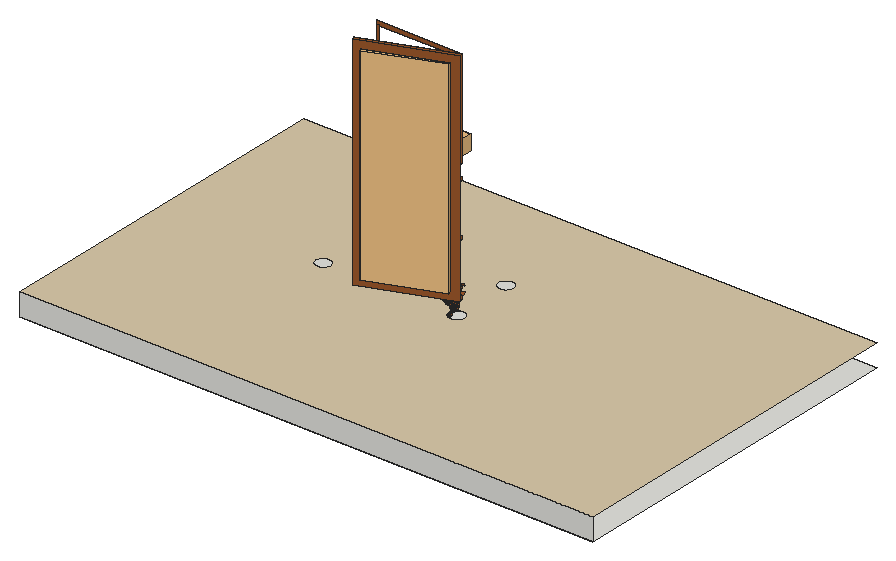
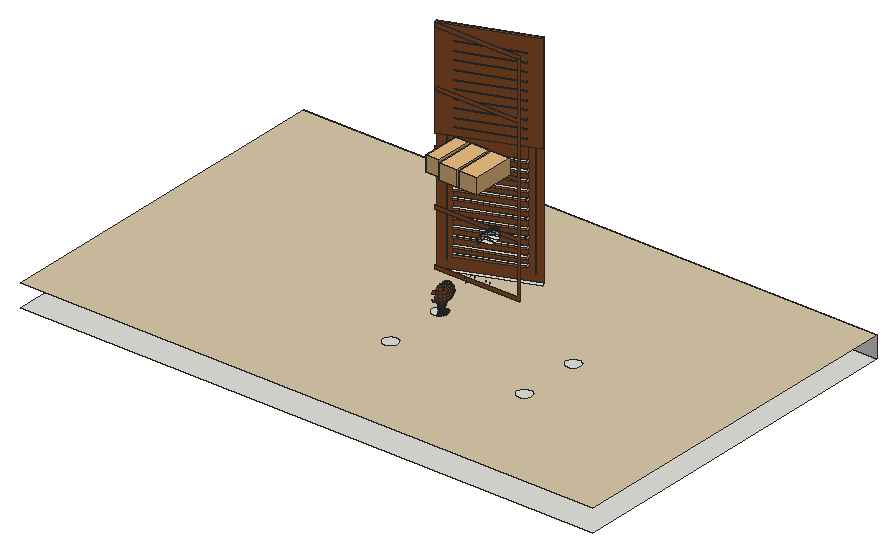
# SketchUp Ruby script. Lengths in inches.
U = 1.inch
M = Sketchup.active_model
def pt(a) = Geom::Point3d.new(a.map { |v| v * U })
def face(e, loops, mat)
  f = e.add_face(loops[0].map { |a| pt(a) })
  loops[1..].each { |l| e.add_face(l.map { |a| pt(a) }).erase! }
  f.material = f.back_material = mat if mat
  f
end
# faces: each face lists its corners as indices into pts; further lists are holes
def faces(e, pts, list, mat = nil) = list.each { |f| face(e, (f[0].is_a?(Array) ? f : [f]).map { |l| l.map { |i| pts[i] } }, mat) }
# xy, xz, yz: faces in a plane at the given z, y or x. An outline is a flat list of corners, or four numbers for a rectangle; further outlines are holes
def ring(l) = l.size == 4 ? [[l[0], l[1]], [l[2], l[1]], [l[2], l[3]], [l[0], l[3]]] : l.each_slice(2).to_a
def flat(e, list, mat, &to3) = list.each { |f| face(e, (f[0].is_a?(Array) ? f : [f]).map { |l| ring(l).map { |u, v| to3.(u, v) } }, mat) }
def xy(e, z, list, mat = nil) = flat(e, list, mat) { |x, y| [x, y, z] }
def xz(e, y, list, mat = nil) = flat(e, list, mat) { |x, z| [x, y, z] }
def yz(e, x, list, mat = nil) = flat(e, list, mat) { |y, z| [x, y, z] }
def lines(e, pts, list) = list.each { |a, b| e.add_line(pt(pts[a]), pt(pts[b])) }
# prism: a flat outline (further loops are holes) pulled along v
def prism(e, loops, v, mat = nil)
  f = face(e, loops, mat); d = Geom::Vector3d.new(v.map { |x| x * U })
  f.pushpull(f.normal.samedirection?(d) ? d.length : -d.length)
end
def box(e, o, s, mat = nil) = prism(e, [[o, [o[0] + s[0], o[1], o[2]], [o[0] + s[0], o[1] + s[1], o[2]], [o[0], o[1] + s[1], o[2]]]], [0, 0, s[2]], mat)
def at(x, y, z, deg = 0) = Geom::Transformation.translation(pt([x, y, z])) * Geom::Transformation.rotation(ORIGIN, Z_AXIS, deg.degrees)
def axes(o, x, y, z) = Geom::Transformation.new([*x, 0, *y, 0, *z, 0, *pt(o).to_a, 1])
def part(name) = M.definitions.add(name)
# library, detail: a bought-in or finely detailed component or shape, given as its bounding box
def library(name, o, s) = part(name).tap { |d| box(d.entities, o, s) }
def detail(e, o, s) = box(e.add_group.entities, o, s)
def put(e, d, t, mat = nil) = e.add_instance(d, t).tap { |i| i.material = mat if mat }
def group(e, t, mat = nil) = e.add_group.tap { |g| g.transformation = t; g.material = mat if mat }.entities
root = M.entities
M.materials.add("[Color K04]").color = [255, 50, 255]
M.materials.add("[Color L16]").color = [102, 0, 51]
M.materials.add("[Color M03]").color = [170, 170, 170]
M.materials.add("[Field Square Tile]").color = [217, 201, 169]
M.materials.add("[Wood Cherry Original]").color = [152, 86, 42]
c1 = library("shoe3",[0,0,0],[5.04,11.41,4.2])
c2 = part("Group\#13")
detail(c2.entities,[0,0,0],[19.875,0.8125,55.92])
c3 = library("Group\#9",[0,0,0],[6.05,17.1,6.94])
xy(root,0,[[118.75,0,274.48,96.25]])
xy(root,6,[[[118.75,0,274.48,96.25],[197.18,64.59,196.64,64.74,196.16,65.02,195.76,65.42,195.49,65.9,195.34,66.44,195.35,67,195.49,67.54,195.77,68.02,196.17,68.41,196.65,68.69,197.19,68.83,197.75,68.83,198.29,68.69,198.77,68.4,199.17,68.01,199.44,67.52,199.59,66.98,199.59,66.42,199.4375,65.89,199.16,65.4,198.76,65.01,198.28,64.73,197.74,64.59],[160.74,64.59,160.2,64.74,159.72,65.02,159.33,65.42,159.05,65.9,158.91,66.44,158.91,67,159.06,67.54,159.34,68.02,159.73,68.41,160.22,68.69,160.76,68.83,161.32,68.83,161.85,68.69,162.34,68.4,162.73,68.01,163.01,67.52,163.15,66.98,163.15,66.42,163,65.89,162.72,65.4,162.32,65.01,161.84,64.73,161.3,64.59],[160.74,47.97,160.2,48.11,159.72,48.4,159.33,48.79,159.05,49.28,158.91,49.82,158.91,50.375,159.06,50.91,159.34,51.4,159.73,51.79,160.22,52.07,160.76,52.21,161.32,52.21,161.85,52.06,162.34,51.78,162.73,51.38,163.01,50.9,163.15,50.36,163.15,49.8,163,49.26,162.72,48.78,162.32,48.39,161.84,48.11,161.3,47.97],[197.18,47.97,196.64,48.11,196.16,48.4,195.76,48.79,195.49,49.28,195.34,49.82,195.35,50.375,195.49,50.91,195.77,51.4,196.17,51.79,196.65,52.07,197.19,52.21,197.75,52.21,198.29,52.06,198.77,51.78,199.17,51.38,199.44,50.9,199.59,50.36,199.59,49.8,199.4375,49.26,199.16,48.78,198.76,48.39,198.28,48.11,197.74,47.97]]],"[Field Square Tile]")
xy(root,6,[[196.64,48.11,196.7,48.25,196.25,48.51,196.16,48.4],[196.16,48.4,196.25,48.51,195.88,48.88,195.76,48.79],[195.76,48.79,195.88,48.88,195.625,49.33,195.49,49.28],[195.49,49.28,195.625,49.33,195.49,49.84,195.34,49.82],[195.34,49.82,195.49,49.84,195.5,50.35,195.35,50.375],
  [195.5,50.35,195.63,50.85,195.49,50.91,195.35,50.375],[195.63,50.85,195.89,51.3,195.77,51.4,195.49,50.91],[195.89,51.3,196.26,51.67,196.17,51.79,195.77,51.4],[196.26,51.67,196.71,51.93,196.65,52.07,196.17,51.79]],"[Wood Cherry Original]")
xy(root,13.08,[[179.8,36.6,179.45,37.53,201.81,46.11,202.17,45.18]])
xy(root,16.73,[[183.07,37.85,198.59,43.81,198.23,44.74,182.72,38.79]],"[Wood Cherry Original]")
xy(root,17.26,[[183.07,37.85,182.72,38.79,198.23,44.74,198.59,43.81]])
xy(root,18.83,[[183.07,37.85,198.59,43.81,198.23,44.74,182.72,38.79]],"[Wood Cherry Original]")
xy(root,19.33,[[183.07,37.85,182.72,38.79,198.23,44.74,198.59,43.81]])
xy(root,21.15,[[183.07,37.85,198.59,43.81,198.23,44.74,182.72,38.79]],"[Wood Cherry Original]")
xy(root,21.65,[[183.07,37.85,182.72,38.79,198.23,44.74,198.59,43.81]])
xy(root,23.48,[[183.07,37.85,198.59,43.81,198.23,44.74,182.72,38.79]],"[Wood Cherry Original]")
xy(root,23.98,[[183.07,37.85,182.72,38.79,198.23,44.74,198.59,43.81]])
xy(root,25.8,[[183.07,37.85,198.59,43.81,198.23,44.74,182.72,38.79]],"[Wood Cherry Original]")
xy(root,26.3,[[183.07,37.85,182.72,38.79,198.23,44.74,198.59,43.81]])
xy(root,28.125,[[183.07,37.85,198.59,43.81,198.23,44.74,182.72,38.79]],"[Wood Cherry Original]")
xy(root,28.59,[[182.89,47.98,182.22,48.5,181.75,49.77,184.52,50.36,184.5,48.98,184,48.21]],"[Color K04]")
xy(root,28.625,[[183.07,37.85,182.72,38.79,198.23,44.74,198.59,43.81]])
xy(root,28.72,[[182.9,48.04,183.97,48.26,184.4375,49,182.27,48.54],[182.27,48.54,184.4375,49,184.46,50.35,181.81,49.78]])
xy(root,30.45,[[183.07,37.85,198.59,43.81,198.23,44.74,182.72,38.79]],"[Wood Cherry Original]")
xy(root,30.95,[[183.07,37.85,182.72,38.79,198.23,44.74,198.59,43.81]])
xy(root,32.78,[[183.07,37.85,198.59,43.81,198.23,44.74,182.72,38.79]],"[Wood Cherry Original]")
xy(root,33.28,[[183.07,37.85,182.72,38.79,198.23,44.74,198.59,43.81]])
xy(root,35.1,[[183.07,37.85,198.59,43.81,198.23,44.74,182.72,38.79]],"[Wood Cherry Original]")
xy(root,35.6,[[183.07,37.85,182.72,38.79,198.23,44.74,198.59,43.81]])
xy(root,37.43,[[183.07,37.85,198.59,43.81,198.23,44.74,182.72,38.79]],"[Wood Cherry Original]")
xy(root,37.93,[[183.07,37.85,182.72,38.79,198.23,44.74,198.59,43.81]])
xy(root,39.75,[[183.07,37.85,198.59,43.81,198.23,44.74,182.72,38.79]],"[Wood Cherry Original]")
xy(root,40.25,[[183.07,37.85,182.72,38.79,198.23,44.74,198.59,43.81]])
xy(root,42.08,[[183.07,37.85,198.59,43.81,198.23,44.74,182.72,38.79]],"[Wood Cherry Original]")
xy(root,42.58,[[183.07,37.85,182.72,38.79,198.23,44.74,198.59,43.81]])
xy(root,47.97,[[183.07,37.85,198.59,43.81,198.23,44.74,182.72,38.79]],"[Wood Cherry Original]")
xy(root,48.47,[[183.07,37.85,182.72,38.79,198.23,44.74,198.59,43.81]])
xy(root,50.29,[[183.07,37.85,198.59,43.81,198.23,44.74,182.72,38.79]],"[Wood Cherry Original]")
xy(root,50.79,[[183.07,37.85,182.72,38.79,198.23,44.74,198.59,43.81]])
xy(root,52.62,[[183.07,37.85,198.59,43.81,198.23,44.74,182.72,38.79]],"[Wood Cherry Original]")
xy(root,53.12,[[183.07,37.85,182.72,38.79,198.23,44.74,198.59,43.81]])
xy(root,54.94,[[183.07,37.85,198.59,43.81,198.23,44.74,182.72,38.79]],"[Wood Cherry Original]")
xy(root,55.44,[[183.07,37.85,182.72,38.79,198.23,44.74,198.59,43.81]])
xy(root,57.27,[[183.07,37.85,198.59,43.81,198.23,44.74,182.72,38.79]],"[Wood Cherry Original]")
xy(root,57.77,[[183.07,37.85,182.72,38.79,198.23,44.74,198.59,43.81]])
xy(root,59.59,[[183.07,37.85,198.59,43.81,198.23,44.74,182.72,38.79]],"[Wood Cherry Original]")
xy(root,60.09,[[183.07,37.85,182.72,38.79,198.23,44.74,198.59,43.81]])
xy(root,61.92,[[183.07,37.85,198.59,43.81,198.23,44.74,182.72,38.79]],"[Wood Cherry Original]")
xy(root,62.42,[[183.07,37.85,182.72,38.79,198.23,44.74,198.59,43.81]])
xy(root,64.24,[[183.07,37.85,198.59,43.81,198.23,44.74,182.72,38.79]],"[Wood Cherry Original]")
xy(root,64.74,[[183.07,37.85,182.72,38.79,198.23,44.74,198.59,43.81]])
xy(root,66.57,[[183.07,37.85,198.59,43.81,198.23,44.74,182.72,38.79]],"[Wood Cherry Original]")
xy(root,67.07,[[183.07,37.85,182.72,38.79,198.23,44.74,198.59,43.81]])
xy(root,68.89,[[183.07,37.85,198.59,43.81,198.23,44.74,182.72,38.79]],"[Wood Cherry Original]")
xy(root,69.39,[[183.07,37.85,182.72,38.79,198.23,44.74,198.59,43.81]])
xy(root,73.08,[[179.8,36.6,202.17,45.18,201.81,46.11,179.45,37.53]],"[Wood Cherry Original]")
xz(root,0,[[118.75,0,274.48,6]])
xz(root,46.11,[[178.85,13.08,201.81,13.08,201.81,14.08,179.35,14.08,179.35,27.58,201.81,27.58,201.81,28.58,179.35,28.58,179.35,42.08,201.81,42.08,201.81,43.08,179.35,43.08,179.35,56.58,201.81,56.58,201.81,57.58,179.35,57.58,179.35,72.08,178.85,72.08],[178.85,72.08,201.81,73.08]],"[Wood Cherry Original]")
yz(root,195.97,[[49.9,8.1,50.29,8.4]],"[Wood Cherry Original]")
yz(root,196.27,[[49.93,6.79,50.25,6.94]],"[Wood Cherry Original]")
p = [[196.34,48.63,6.03],[196.25,48.51,6],[196.7,48.25,6],[196.76,48.39,6.03],[196.43,48.75,6.08],[196.81,48.52,6.08],
  [196,48.97,6.03],[195.88,48.88,6],[196.12,49.06,6.08],[195.76,49.39,6.03],[195.625,49.33,6],[195.9,49.44,6.08],
  [195.64,49.85,6.03],[195.49,49.84,6],[195.78,49.87,6.08],[195.64,50.33,6.03],[195.5,50.35,6],[195.78,50.32,6.08],
  [195.77,50.8,6.03],[195.63,50.85,6],[195.9,50.74,6.08],[196.125,51.125,6.08],[196.01,51.21,6.03],[195.89,51.3,6],
  [196.4375,51.4375,6.08],[196.35,51.55,6.03],[196.26,51.67,6],[196.82,51.66,6.08],[196.77,51.79,6.03],[196.71,51.93,6],
  [196.51,48.85,6.16],[196.86,48.64,6.16],[196.22,49.14,6.16],[196.02,49.49,6.16],[195.91,49.89,6.16],[195.91,50.3,6.16],
  [196.02,50.69,6.16],[196.23,51.05,6.16],[196.52,51.33,6.16],[196.87,51.54,6.16],[196.58,48.94,6.25],[196.91,48.75,6.25],
  [196.3125,49.21,6.25],[196.125,49.54,6.25],[196.03,49.9,6.25],[196.03,50.28,6.25],[196.13,50.65,6.25],[196.32,50.97,6.25],
  [196.59,51.24,6.25],[196.92,51.43,6.25],[196.64,49.02,6.37],[196.94,48.84,6.37],[196.39,49.27,6.37],[196.21,49.57,6.37],
  [196.12,49.92,6.37],[196.125,50.27,6.37],[196.22,50.61,6.37],[196.39,50.92,6.37],[196.65,51.16,6.37],[196.95,51.34,6.37],
  [196.68,49.08,6.5],[196.97,48.91,6.5],[196.45,49.3125,6.5],[196.28,49.6,6.5],[196.2,49.93,6.5],[196.2,50.26,6.5],
  [196.29,50.58,6.5],[196.45,50.87,6.5],[196.69,51.1,6.5],[196.98,51.27,6.5],[196.49,49.34,6.64],[196.71,49.12,6.64],
  [196.33,49.62,6.64],[196.25,49.93,6.64],[196.25,50.25,6.64],[196.33,50.5625,6.64],[196.49,50.84,6.64],[196.72,51.0625,6.64],
  [196.51,49.36,6.79],[196.73,49.14,6.79],[196.35,49.63,6.79],[196.27,49.93,6.79],[196.27,50.25,6.79],[196.36,50.55,6.79],
  [196.51,50.82,6.79],[196.74,51.04,6.79],[196.51,49.36,6.94],[196.73,49.14,6.94],[196.35,49.63,6.94],[196.27,49.93,6.94],
  [196.36,50.55,6.94],[196.27,50.25,6.94],[196.51,50.82,6.94],[196.74,51.04,6.94],[196.49,49.34,7.09],[196.71,49.12,7.09],
  [196.33,49.62,7.09],[196.25,49.93,7.09],[196.25,50.25,7.09],[196.33,50.5625,7.09],[196.49,50.84,7.09],[196.72,51.06,7.09],
  [196.45,49.3125,7.23],[196.68,49.07,7.23],[196.28,49.6,7.23],[196.2,49.92,7.23],[196.2,50.26,7.23],[196.28,50.58,7.23],
  [196.45,50.87,7.23],[196.69,51.11,7.23],[196.61,48.99,7.51],[196.97,48.91,7.23],[196.93,48.8,7.51],[196.36,49.24,7.51],
  [196.18,49.56,7.51],[196.09,49.91,7.51],[196.09,50.27,7.51],[196.18,50.625,7.51],[196.36,50.9375,7.51],[196.62,51.19,7.51],
  [196.9375,51.375,7.51],[196.98,51.27,7.23],[196.57,48.93,7.8],[196.9,48.73,7.8],[196.3,49.2,7.8],[196.11,49.53,7.8],
  [196.01,49.9,7.8],[196.01,50.28,7.8],[196.11,50.65,7.8],[196.3,50.98,7.8],[196.58,51.25,7.8],[196.91,51.45,7.8],
  [196.54,48.89,8.1],[196.88,48.7,8.1],[196.27,49.17,8.1],[196.07,49.52,8.1],[195.97,49.9,8.1],[195.97,50.29,8.1],
  [196.08,50.67,8.1],[196.27,51.01,8.1],[196.55,51.29,8.1],[196.89,51.48,8.1],[196.54,48.89,8.4],[196.88,48.69,8.4],
  [196.26,49.17,8.4],[196.07,49.51,8.4],[195.97,49.9,8.4],[196.07,50.67,8.4],[195.97,50.29,8.4],[196.27,51.01,8.4],
  [196.55,51.29,8.4],[196.89,51.48,8.4],[196.5625,48.92,8.7],[196.9,48.73,8.7],[196.29,49.19,8.7],[196.1,49.53,8.7],
  [196,49.9,8.7],[196,50.29,8.7],[196.1,50.66,8.7],[196.3,50.99,8.7],[196.57,51.26,8.7],[196.91,51.45,8.7],
  [196.61,48.98,8.99],[196.92,48.79,8.99],[196.35,49.24,8.99],[196.16,49.55,8.99],[196.07,49.91,8.99],[196.07,50.28,8.99],
  [196.17,50.63,8.99],[196.35,50.95,8.99],[196.61,51.21,8.99],[196.93,51.39,8.99],[196.18,48.42,9.21],[196.65,48.14,9.21],
  [195.79,48.81,9.21],[195.52,49.29,9.21],[195.375,49.82,9.21],[195.375,50.37,9.21],[195.52,50.9,9.21],[195.8,51.375,9.21],
  [196.1875,51.76,9.21],[196.67,52.04,9.21],[195.82,47.96,9.66],[196.43,47.61,9.66],[195.33,48.46,9.66],[194.98,49.07,9.66],
  [194.8,49.75,9.66],[194.8,50.45,9.66],[194.99,51.125,9.66],[195.34,51.73,9.66],[195.84,52.23,9.66],[196.45,52.57,9.66],
  [196.28,47.26,10.28],[197.1,47.42,9.66],[197.05,47.05,10.28],[195.59,47.66,10.28],[195.02,48.23,10.28],[194.63,48.92,10.28],
  [194.42,49.7,10.28],[194.43,50.5,10.28],[194.64,51.27,10.28],[195.04,51.96,10.28],[195.61,52.53,10.28],[196.3,52.93,10.28],
  [197.08,53.13,10.28],[197.125,52.75,9.66],[196.23,47.14,11],[197.04,46.92,11],[195.51,47.56,11],[194.92,48.15,11],
  [194.5,48.875,11],[194.29,49.68,11],[194.29,50.52,11],[194.51,51.32,11],[194.93,52.04,11],[195.53,52.63,11],
  [196.25,53.05,11],[196.28,47.26,11.72],[197.05,47.05,11.72],[195.59,47.66,11.72],[195.02,48.23,11.72],[194.63,48.92,11.72],
  [194.42,49.7,11.72],[194.43,50.5,11.72],[194.64,51.27,11.72],[195.04,51.96,11.72],[195.61,52.53,11.72],[196.3,52.93,11.72],
  [196.43,47.61,12.34],[197.1,47.42,12.34],[195.82,47.96,12.34],[195.33,48.46,12.34],[194.98,49.07,12.34],[194.8,49.75,12.34],
  [194.8,50.45,12.34],[194.99,51.125,12.34],[195.34,51.73,12.34],[195.84,52.23,12.34],[196.45,52.57,12.34],[197.125,52.75,12.34],
  [197.08,53.13,11.72],[196.18,48.42,12.79],[196.65,48.14,12.79],[195.79,48.81,12.79],[195.52,49.29,12.79],[195.375,49.82,12.79],
  [195.375,50.37,12.79],[195.52,50.9,12.79],[195.8,51.375,12.79],[196.1875,51.76,12.79],[196.67,52.04,12.79],[196.61,48.98,13.01],
  [196.92,48.79,13.01],[196.35,49.24,13.01],[196.16,49.55,13.01],[196.07,49.91,13.01],[196.07,50.28,13.01],[196.17,50.63,13.01],
  [196.35,50.95,13.01],[196.61,51.21,13.01],[196.93,51.39,13.01],[196.93,49.68,12.97],[197.05,49.56,12.97],[196.84,49.83,12.97],
  [196.8,50,12.97],[196.8,50.18,12.97],[196.85,50.35,12.97],[196.93,50.5,12.97],[197.06,50.62,12.97],[179.8,36.6,13.08],
  [202.17,45.18,13.08],[202.17,45.18,73.08],[179.8,36.6,73.08],[198.59,43.81,16.73],[183.07,37.85,16.73],[183.07,37.85,17.26],
  [183.07,37.85,18.83],[183.07,37.85,19.33],[183.07,37.85,21.15],[183.07,37.85,21.65],[183.07,37.85,23.48],[183.07,37.85,23.98],
  [183.07,37.85,25.8],[183.07,37.85,26.3],[183.07,37.85,28.125],[183.07,37.85,28.625],[183.07,37.85,30.45],[183.07,37.85,30.95],
  [183.07,37.85,32.78],[183.07,37.85,33.28],[183.07,37.85,35.1],[183.07,37.85,35.6],[183.07,37.85,37.43],[183.07,37.85,37.93],
  [183.07,37.85,39.75],[183.07,37.85,40.25],[183.07,37.85,42.08],[183.07,37.85,42.58],[183.07,37.85,47.97],[183.07,37.85,48.47],
  [183.07,37.85,50.29],[183.07,37.85,50.79],[183.07,37.85,52.62],[183.07,37.85,53.12],[183.07,37.85,54.94],[183.07,37.85,55.44],
  [183.07,37.85,57.27],[183.07,37.85,57.77],[183.07,37.85,59.59],[183.07,37.85,60.09],[183.07,37.85,61.92],[183.07,37.85,62.42],
  [183.07,37.85,64.24],[183.07,37.85,64.74],[183.07,37.85,66.57],[183.07,37.85,67.07],[183.07,37.85,68.89],[183.07,37.85,69.39],
  [198.59,43.81,69.39],[198.59,43.81,68.89],[198.59,43.81,67.07],[198.59,43.81,66.57],[198.59,43.81,64.74],[198.59,43.81,64.24],
  [198.59,43.81,62.42],[198.59,43.81,61.92],[198.59,43.81,60.09],[198.59,43.81,59.59],[198.59,43.81,57.77],[198.59,43.81,57.27],
  [198.59,43.81,55.44],[198.59,43.81,54.94],[198.59,43.81,53.12],[198.59,43.81,52.62],[198.59,43.81,50.79],[198.59,43.81,50.29],
  [198.59,43.81,48.47],[198.59,43.81,47.97],[198.59,43.81,42.58],[198.59,43.81,42.08],[198.59,43.81,40.25],[198.59,43.81,39.75],
  [198.59,43.81,37.93],[198.59,43.81,37.43],[198.59,43.81,35.6],[198.59,43.81,35.1],[198.59,43.81,33.28],[198.59,43.81,32.78],
  [198.59,43.81,30.95],[198.59,43.81,30.45],[198.59,43.81,28.625],[198.59,43.81,28.125],[198.59,43.81,26.3],[198.59,43.81,25.8],
  [198.59,43.81,23.98],[198.59,43.81,23.48],[198.59,43.81,21.65],[198.59,43.81,21.15],[198.59,43.81,19.33],[198.59,43.81,18.83],
  [198.59,43.81,17.26],[182.72,38.79,16.73],[182.72,38.79,17.26],[188.82,52.19,17.8125],[188.82,52.2,17.86],[188.78,52.07,18],
  [188.78,51.96,16.99],[188.78,51.95,16.83],[188.78,51.97,16.9],[188.78,52.09,18.17],[188.82,52.23,18.19],[188.84,52.25,17.82],
  [183.02,51.03,18.4],[182.99,51.04,18.23],[183.02,51.02,18.23],[184.19,51.03,18.4],[184.1875,51.02,18.23],[184.22,51.04,18.23],
  [186.99,51.03,18.4],[186.96,51.04,18.23],[186.99,51.02,18.23],[188.15,51.03,18.4],[188.16,51.02,18.23],[188.1875,51.04,18.23],
  [182.72,38.79,18.83],[182.72,38.79,19.33],[182.72,38.79,21.15],[182.72,38.79,21.65],[182.72,38.79,23.48],[182.72,38.79,23.98],
  [182.72,38.79,25.8],[182.72,38.79,26.3],[182.72,38.79,28.125],[182.72,38.79,28.625],[182.89,47.98,28.59],[182.87,47.89,28.67],
  [182.13,48.48,28.67],[184,48.21,28.59],[184.05,48.14,28.67],[184.5,48.98,28.59],[184.59,49,28.67],[184.52,50.36,28.59],
  [184.6,50.375,28.67],[181.58,51.11,28.65],[184.32,51.48,28.65],[184.18,52.65,28.74],[184.1,52.64,28.66],[184.07,53.66,28.58],
  [182.87,47.89,28.96],[184.05,48.14,28.96],[182.9,48.03,29.63],[182.9,48.04,28.72],[182.27,48.54,28.72],[183.97,48.26,29.63],
  [183.97,48.26,28.72],[184.59,49,28.96],[184.375,49.1,29.625],[184.4375,49,28.72],[184.38,50.39,29.53],[184.46,50.35,28.72],
  [184.6,50.375,28.96],[181.63,51.12,28.78],[181.81,49.78,28.72],[184.27,51.47,28.78],[184.29,51.46,29.46],[184.4,51.49,28.73],
  [184.4,51.49,28.96],[181.45,52.22,28.66],[184.18,52.65,28.96],[184.05,52.64,28.79],[181.51,52.23,28.79],[184.15,52.65,29.4],
  [184.17,53.7,29.36],[182.86,47.9,29.65],[184.06,48.15,29.65],[184.51,49.0625,29.65],[184.52,50.4,29.55],[184.43,51.47,29.47],
  [184.29,52.66,29.38],[184.3125,53.69,29.34],[184.19,52.7,29.96],[184.33,52.7,29.97],[184.22,53.7,29.89],[184.36,53.7,29.89],
  [184.21,50.36,30.17],[184.2,51.51,30.06],[184.34,51.52,30.09],[182.14,48.51,29.65],[182.9,48.04,30.32],[183.8,48.21,30.32],
  [182.93,48.17,30.28],[182.26,48.59,29.63],[183.73,48.32,30.27],[184.25,49.08,30.32],[184.13,49.11,30.25],[184.34,50.37,30.23],
  [184.13,52.74,30.47],[184.27,52.74,30.55],[184.01,51.56,30.57],[184.11,51.56,30.68],[183.9,50.41,30.65],[183.97,50.41,30.79],
  [182.27,48.6,30.32],[182.93,48.29,30.9],[183.51,48.4,30.9],[182.97,48.38,30.78],[182.38,48.68,30.28],[183.47,48.48,30.77],
  [183.77,49.23,30.9],[183.72,49.25,30.76],[182.6,48.79,30.78],[182.72,38.79,30.45],[182.72,38.79,30.95],[184.04,51.56,30.65],
  [184.1875,52.75,30.54],[183.91,50.41,30.74],[183.72,49.25,30.84],[182.58,48.78,30.86],[182.95,48.35,30.87],[183.47,48.45,30.86],
  [182.51,48.74,30.9],[182.72,38.79,32.78],[182.72,38.79,33.28],[182.72,38.79,35.1],[182.72,38.79,35.6],[182.72,38.79,37.43],
  [182.72,38.79,37.93],[182.72,38.79,39.75],[182.72,38.79,40.25],[182.72,38.79,42.08],[182.72,38.79,42.58],[201.81,46.11,56.58],
  [201.81,46.11,46.26],[179.45,37.53,46.26],[179.45,37.53,73.08],[201.81,46.11,73.08],[201.81,46.11,72.08],[201.81,46.11,57.58],
  [182.72,38.79,69.39],[182.72,38.79,68.89],[198.23,44.74,68.89],[198.23,44.74,69.39],[182.72,38.79,67.07],[182.72,38.79,66.57],
  [198.23,44.74,66.57],[198.23,44.74,67.07],[182.72,38.79,64.74],[182.72,38.79,64.24],[198.23,44.74,64.24],[198.23,44.74,64.74],
  [182.72,38.79,62.42],[182.72,38.79,61.92],[198.23,44.74,61.92],[198.23,44.74,62.42],[182.72,38.79,60.09],[182.72,38.79,59.59],
  [198.23,44.74,59.59],[198.23,44.74,60.09],[182.72,38.79,57.77],[182.72,38.79,57.27],[198.23,44.74,57.27],[198.23,44.74,57.77],
  [182.72,38.79,55.44],[182.72,38.79,54.94],[198.23,44.74,54.94],[198.23,44.74,55.44],[182.72,38.79,53.12],[182.72,38.79,52.62],
  [198.23,44.74,52.62],[198.23,44.74,53.12],[182.72,38.79,50.79],[182.72,38.79,50.29],[198.23,44.74,50.29],[198.23,44.74,50.79],
  [182.72,38.79,48.47],[182.72,38.79,47.97],[198.23,44.74,47.97],[198.23,44.74,48.47]]
faces(root,p,[[0,1,2,3],[4,0,3,5],[6,7,1,0],[8,6,0,4],[9,10,7,6],[11,9,6,8],[12,13,10,9],[14,12,9,11],
  [15,16,13,12],[17,15,12,14],[18,19,16,15],[20,18,15,17],[21,22,18,20],[22,23,19,18],[24,25,22,21],[25,26,23,22],
  [27,28,25,24],[28,29,26,25],[30,4,5,31],[32,8,4,30],[33,11,8,32],[34,14,11,33],[35,17,14,34],[36,20,17,35],
  [37,21,20,36],[38,24,21,37],[39,27,24,38],[40,30,31,41],[42,32,30,40],[43,33,32,42],[44,34,33,43],[45,35,34,44],
  [46,36,35,45],[47,37,36,46],[48,38,37,47],[49,39,38,48],[50,40,41,51],[52,42,40,50],[53,43,42,52],[54,44,43,53],
  [55,45,44,54],[56,46,45,55],[57,47,46,56],[58,48,47,57],[59,49,48,58],[60,50,51,61],[62,52,50,60],[63,53,52,62],
  [64,54,53,63],[65,55,54,64],[66,56,55,65],[67,57,56,66],[68,58,57,67],[69,59,58,68],[70,62,60,71],[72,63,62,70],
  [73,64,63,72],[74,65,64,73],[75,66,65,74],[76,67,66,75],[77,68,67,76],[78,70,71,79],[80,72,70,78],[81,73,72,80],
  [82,74,73,81],[83,75,74,82],[84,76,75,83],[85,77,76,84],[86,78,79,87],[88,80,78,86],[89,81,80,88],[90,83,82,91],
  [92,84,83,90],[93,85,84,92],[94,86,87,95],[96,88,86,94],[97,89,88,96],[98,91,89,97],[99,90,91,98],[100,92,90,99],
  [101,93,92,100],[102,94,95,103],[104,96,94,102],[105,97,96,104],[106,98,97,105],[107,99,98,106],[108,100,99,107],[109,101,100,108],
  [110,103,111,112],[113,102,103,110],[114,104,102,113],[115,105,104,114],[116,106,105,115],[117,107,106,116],[118,108,107,117],[119,109,108,118],
  [120,121,109,119],[122,110,112,123],[124,113,110,122],[125,114,113,124],[126,115,114,125],[127,116,115,126],[128,117,116,127],[129,118,117,128],
  [130,119,118,129],[131,120,119,130],[132,122,123,133],[134,124,122,132],[135,125,124,134],[136,126,125,135],[137,127,126,136],[138,128,127,137],
  [139,129,128,138],[140,130,129,139],[141,131,130,140],[142,132,133,143],[144,134,132,142],[145,135,134,144],[146,136,135,145],[147,138,137,148],
  [149,139,138,147],[150,140,139,149],[151,141,140,150],[152,142,143,153],[154,144,142,152],[155,145,144,154],[156,146,145,155],[157,148,146,156],
  [158,147,148,157],[159,149,147,158],[160,150,149,159],[161,151,150,160],[162,152,153,163],[164,154,152,162],[165,155,154,164],[166,156,155,165],
  [167,157,156,166],[168,158,157,167],[169,159,158,168],[170,160,159,169],[171,161,160,170],[172,162,163,173],[174,164,162,172],[175,165,164,174],
  [176,166,165,175],[177,167,166,176],[178,168,167,177],[179,169,168,178],[180,170,169,179],[181,171,170,180],[182,172,173,183],[184,174,172,182],
  [185,175,174,184],[186,176,175,185],[187,177,176,186],[188,178,177,187],[189,179,178,188],[190,180,179,189],[191,181,180,190],[192,183,193,194],
  [195,182,183,192],[196,184,182,195],[197,185,184,196],[198,186,185,197],[199,187,186,198],[200,188,187,199],[201,189,188,200],[202,190,189,201],
  [203,191,190,202],[204,205,191,203],[206,192,194,207],[208,195,192,206],[209,196,195,208],[210,197,196,209],[211,198,197,210],[212,199,198,211],
  [213,200,199,212],[214,201,200,213],[215,202,201,214],[216,203,202,215],[217,206,207,218],[219,208,206,217],[220,209,208,219],[221,210,209,220],
  [222,211,210,221],[223,212,211,222],[224,213,212,223],[225,214,213,224],[226,215,214,225],[227,216,215,226],[228,217,218,229],[230,219,217,228],
  [231,220,219,230],[232,221,220,231],[233,222,221,232],[234,223,222,233],[235,224,223,234],[236,225,224,235],[237,226,225,236],[238,227,226,237],
  [239,240,227,238],[241,230,228,242],[243,231,230,241],[244,232,231,243],[245,233,232,244],[246,234,233,245],[247,235,234,246],[248,236,235,247],
  [249,237,236,248],[250,238,237,249],[251,241,242,252],[253,243,241,251],[254,244,243,253],[255,245,244,254],[256,246,245,255],[257,247,246,256],
  [258,248,247,257],[259,249,248,258],[260,250,249,259],[261,253,251,262],[263,254,253,261],[264,255,254,263],[265,256,255,264],[266,257,256,265],
  [267,258,257,266],[268,259,258,267],[[269,270,271,272],[273,274,275,276,277,278,279,280,281,282,283,284,285,286,287,288,289,290,291,292,293,294,295,296,297,298,299,300,301,302,303,304,305,306,307,308,309,310,311,312,313,314,315,316,317,318,319,320,321,322,323,324,325,326,327,328,329,330,331,332,333,334,335,336,337,338,339,340,341,342,343,344,345,346,347,348,349,350,351,352,353,354,355,356,357,358,359,360]],[360,359,276,275],[358,357,278,277],[356,355,280,279],[354,353,282,281],[352,351,284,283],
  [350,349,286,285],[348,347,288,287],[346,345,290,289],[344,343,292,291],[342,341,294,293],[340,339,296,295],[298,297,338,337],[[491,492,493,494,495,496,497],[498,499,500,501],[502,503,504,505],[506,507,508,509],[510,511,512,513],[514,515,516,517],[518,519,520,521],[522,523,524,525],[526,527,528,529],[530,531,532,533],[534,535,536,537]],
  [336,335,300,299],[334,333,302,301],[332,331,304,303],[330,329,306,305],[328,327,308,307],[326,325,310,309],[324,323,312,311],[322,321,314,313],
  [320,319,316,315]],"[Wood Cherry Original]")
faces(root,p,[[275,274,361,362],[363,364,365,366,367,368],[364,365,369,370,371],[371,363,364],[372,373,374],[375,376,377],[378,379,380],[381,382,383],
  [277,276,384,385],[279,278,386,387],[281,280,388,389],[283,282,390,391],[285,284,392,393],[410,411,412],[410,413,414,411],[414,413,416],
  [416,417,414],[417,416,418],[418,419,417],[421,422,419],[419,423,421],[424,423,419],[419,418,424],[423,429,430,421],
  [431,429,423],[423,424,431],[429,431,432],[440,431,424],[431,440,442],[444,418,416],[418,444,445],[445,424,418],
  [424,445,440],[450,410,451],[410,450,452],[452,413,410],[413,452,454],[454,416,413],[416,454,444],[456,440,445],
  [458,445,444],[445,458,456],[460,444,454],[444,460,458],[465,450,466],[450,465,467],[467,452,450],[452,467,469],
  [469,454,452],[466,470,465],[454,469,460],[287,286,471,472],[458,473,474],[474,456,458],[474,473,459],[459,457,474],
  [460,475,473],[473,475,461],[473,458,460],[461,459,473],[469,476,475],[475,476,468],[475,460,469],[468,461,475],
  [470,477,478],[478,465,470],[465,478,479],[479,467,465],[467,479,476],[476,479,464],[464,468,476],[476,469,467],
  [478,477,480],[480,463,478],[479,478,463],[463,464,479],[289,288,481,482],[291,290,483,484],[293,292,485,486],[295,294,487,488],
  [297,296,489,490],[299,298,535,534],[301,300,531,530],[303,302,527,526],[305,304,523,522],[307,306,519,518],[309,308,515,514],[311,310,511,510],
  [313,312,507,506],[315,314,503,502],[317,316,499,498]])
faces(root,p,[[394,395,396],[394,397,398,395],[398,397,399],[399,400,398],[400,399,401],[401,402,400],[403,404,401],[402,401,404],
  [405,406,407],[408,395,398,409],[409,398,400,415],[415,400,402,420],[404,425,402],[420,402,425,426],[404,403,427,406],[406,405,425],
  [425,404,406],[426,425,405,428],[433,408,409,434],[435,434,409],[409,415,435],[436,435,415],[415,420,436],[420,426,437],
  [437,436,420],[426,428,438],[438,437,426],[439,438,428],[437,438,441],[443,441,438],[436,437,446],[441,446,437],
  [447,433,448],[449,448,433],[433,434,449],[453,449,434],[434,435,453],[455,453,435],[435,436,455],[446,455,436],
  [446,441,457],[455,446,459],[457,459,446],[453,455,461],[459,461,455],[462,448,463],[464,463,448],[448,449,464],
  [468,464,449],[449,453,468],[461,468,453]],"[Color K04]")
put(root,c1,axes([181.64,57.22,43.08],[0.97384,0,0],[0,-0.97384,0],[0,0,0.97384]),"[Color L16]")
put(root,c1,axes([191.92,57.22,43.08],[-0.97384,0,0],[0,-0.97384,0],[0,0,0.97384]),"[Color L16]")
put(root,c2,at(181.85,36.51,15.1,21),"[Wood Cherry Original]")
put(root,c3,axes([192.7,46.11,43.08],[0.5865,0,0],[0,0.5865,0],[0,0,0.5865]),"[Color M03]")
